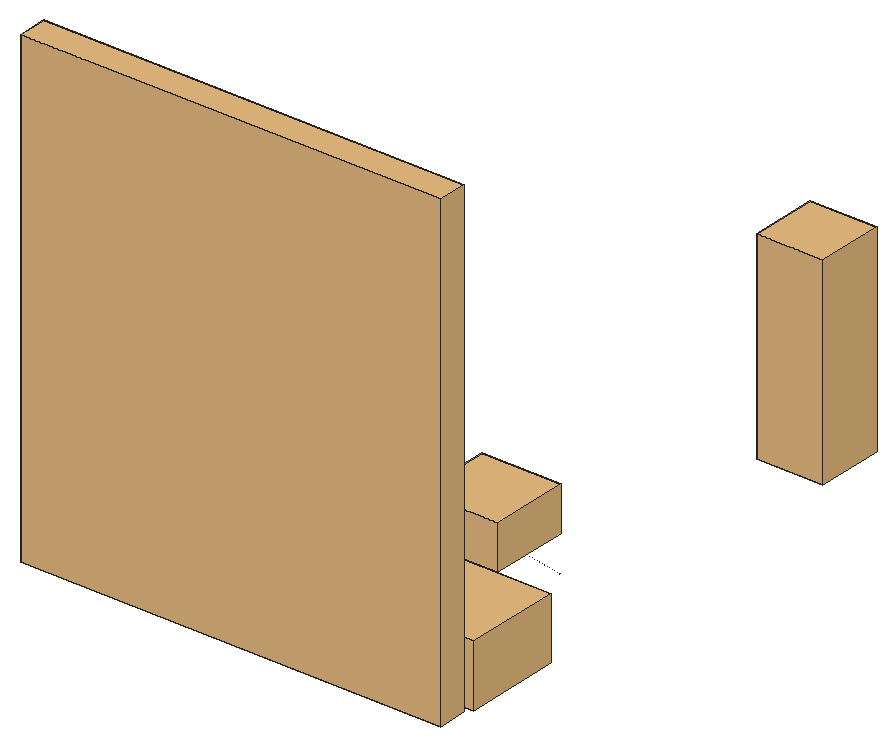
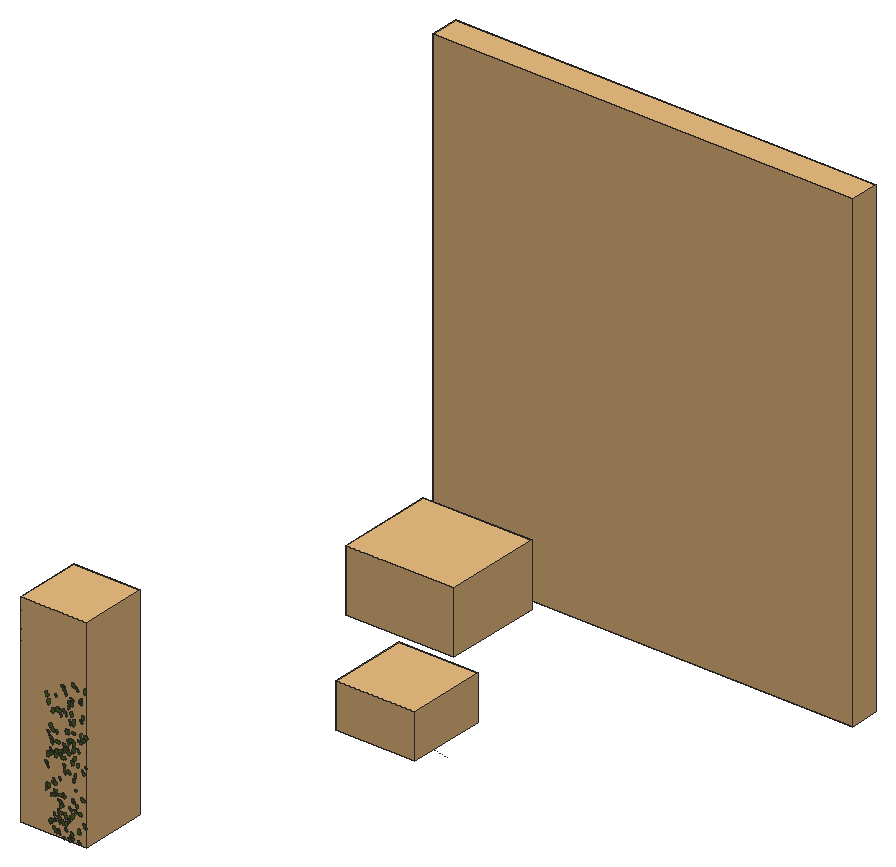
# SketchUp Ruby script. Lengths in inches.
U = 1.inch
M = Sketchup.active_model
def pt(a) = Geom::Point3d.new(a.map { |v| v * U })
def face(e, loops, mat)
  f = e.add_face(loops[0].map { |a| pt(a) })
  loops[1..].each { |l| e.add_face(l.map { |a| pt(a) }).erase! }
  f.material = f.back_material = mat if mat
  f
end
# faces: each face lists its corners as indices into pts; further lists are holes
def faces(e, pts, list, mat = nil) = list.each { |f| face(e, (f[0].is_a?(Array) ? f : [f]).map { |l| l.map { |i| pts[i] } }, mat) }
# xy, xz, yz: faces in a plane at the given z, y or x. An outline is a flat list of corners, or four numbers for a rectangle; further outlines are holes
def ring(l) = l.size == 4 ? [[l[0], l[1]], [l[2], l[1]], [l[2], l[3]], [l[0], l[3]]] : l.each_slice(2).to_a
def flat(e, list, mat, &to3) = list.each { |f| face(e, (f[0].is_a?(Array) ? f : [f]).map { |l| ring(l).map { |u, v| to3.(u, v) } }, mat) }
def xy(e, z, list, mat = nil) = flat(e, list, mat) { |x, y| [x, y, z] }
def xz(e, y, list, mat = nil) = flat(e, list, mat) { |x, z| [x, y, z] }
def yz(e, x, list, mat = nil) = flat(e, list, mat) { |y, z| [x, y, z] }
def lines(e, pts, list) = list.each { |a, b| e.add_line(pt(pts[a]), pt(pts[b])) }
# prism: a flat outline (further loops are holes) pulled along v
def prism(e, loops, v, mat = nil)
  f = face(e, loops, mat); d = Geom::Vector3d.new(v.map { |x| x * U })
  f.pushpull(f.normal.samedirection?(d) ? d.length : -d.length)
end
def box(e, o, s, mat = nil) = prism(e, [[o, [o[0] + s[0], o[1], o[2]], [o[0] + s[0], o[1] + s[1], o[2]], [o[0], o[1] + s[1], o[2]]]], [0, 0, s[2]], mat)
def at(x, y, z, deg = 0) = Geom::Transformation.translation(pt([x, y, z])) * Geom::Transformation.rotation(ORIGIN, Z_AXIS, deg.degrees)
def axes(o, x, y, z) = Geom::Transformation.new([*x, 0, *y, 0, *z, 0, *pt(o).to_a, 1])
def part(name) = M.definitions.add(name)
# library, detail: a bought-in or finely detailed component or shape, given as its bounding box
def library(name, o, s) = part(name).tap { |d| box(d.entities, o, s) }
def detail(e, o, s) = box(e.add_group.entities, o, s)
def put(e, d, t, mat = nil) = e.add_instance(d, t).tap { |i| i.material = mat if mat }
def group(e, t, mat = nil) = e.add_group.tap { |g| g.transformation = t; g.material = mat if mat }.entities
root = M.entities
M.materials.add("[Color M00]1").color = [208, 208, 208]
M.materials.add("[Vegetation Blur 03]").color = [83, 114, 18]
c1 = library("Group\#44",[0,0,-8.125],[130,9,146])
c2 = library("Potted plant",[-17.58,-15.45,-0.53],[33.42,30.09,19.21])
c3 = library("07",[-18.99,-18.99,0],[37.98,37.98,14.32])
c4 = library("Group1\#1",[-13.35,12.45,0],[13.31,13.31,40.49])
c5 = part("ivy")
xy(c5.entities,0,[[0.782,0,0.786,0,0.787,0.005,0.789,0.009,0.821,0.072,0.875,0.147,1.001,0.272,1.073,0.331,1.137,0.363,1.178,0.379,1.223,0.384,1.272,0.383,1.311,0.374,1.36,0.355,1.399,0.334,1.491,0.285,1.541,0.244,1.583,0.199,1.617,0.15,1.64,0.128,1.662,0.115,1.717,0.105,1.745,0.093,1.784,0.054,1.819,0.057,1.854,0.064,1.882,0.075,1.896,0.074,1.91,0.071,1.937,0.063,1.964,0.053,1.99,0.038,2.016,0.015,2.034,0.002,2.04,0,2.038,0.003,2.036,0.007,2.033,0.038,2.036,0.068,2.045,0.1,2.055,0.116,2.064,0.123,2.077,0.129,2.088,0.129,2.106,0.132,2.118,0.13,2.179,0.132,2.207,0.133,2.225,0.133,2.242,0.138,2.22,0.162,2.207,0.186,2.206,0.213,2.212,0.236,2.228,0.262,2.247,0.274,2.298,0.283,2.355,0.294,2.37,0.296,2.376,0.295,2.377,0.3,2.377,0.303,2.385,0.329,2.411,0.37,2.426,0.392,2.449,0.407,2.511,0.426,2.561,0.444,2.619,0.466,2.589,0.469,2.561,0.476,2.501,0.5,2.449,0.516,2.424,0.523,2.401,0.535,2.377,0.556,2.372,0.568,2.36,0.575,2.268,0.586,2.225,0.592,2.207,0.599,2.194,0.61,2.143,0.65,2.13,0.664,2.122,0.682,2.123,0.7,2.13,0.719,2.148,0.75,2.17,0.781,2.195,0.807,2.221,0.828,2.284,0.874,2.291,0.88,2.288,0.887,2.276,0.9,2.267,0.916,2.265,0.933,2.273,0.967,2.292,1.002,2.313,1.03,2.334,1.054,2.348,1.067,2.358,1.074,2.363,1.076,2.362,1.081,2.35,1.094,2.347,1.11,2.35,1.143,2.359,1.18,2.385,1.254,2.415,1.324,2.448,1.393,2.45,1.4,2.446,1.398,2.44,1.394,2.427,1.383,2.402,1.36,2.376,1.339,2.345,1.324,2.305,1.309,2.282,1.303,2.273,1.306,2.245,1.294,2.212,1.287,2.187,1.291,2.163,1.301,2.142,1.316,2.134,1.327,2.124,1.325,2.09,1.292,2.053,1.259,2.014,1.234,1.973,1.215,1.954,1.21,1.931,1.208,1.909,1.212,1.893,1.22,1.879,1.233,1.872,1.248,1.867,1.281,1.864,1.319,1.821,1.258,1.773,1.197,1.726,1.141,1.698,1.121,1.679,1.116,1.666,1.117,1.647,1.122,1.632,1.129,1.62,1.141,1.617,1.154,1.617,1.219,1.621,1.254,1.623,1.268,1.623,1.281,1.618,1.314,1.606,1.346,1.603,1.375,1.607,1.403,1.603,1.467,1.599,1.499,1.605,1.525,1.614,1.552,1.629,1.577,1.635,1.589,1.629,1.587,1.618,1.582,1.596,1.566,1.581,1.556,1.568,1.552,1.557,1.55,1.545,1.553,1.531,1.562,1.522,1.572,1.504,1.591,1.486,1.611,1.474,1.631,1.457,1.666,1.455,1.684,1.457,1.698,1.452,1.715,1.444,1.728,1.424,1.754,1.419,1.772,1.423,1.786,1.434,1.819,1.444,1.848,1.446,1.855,1.44,1.861,1.43,1.867,1.386,1.904,1.349,1.948,1.326,1.973,1.31,1.995,1.288,2.048,1.284,2.153,1.287,2.254,1.284,2.255,1.282,2.253,1.278,2.247,1.274,2.237,1.266,2.216,1.226,2.125,1.208,2.076,1.184,2.033,1.155,1.984,1.135,1.942,1.111,1.899,1.083,1.861,1.053,1.85,1.059,1.83,1.061,1.809,1.056,1.79,1.049,1.767,1.04,1.749,1.018,1.733,0.994,1.726,0.942,1.734,0.95,1.6875,0.944,1.645,0.932,1.608,0.911,1.585,0.881,1.58,0.854,1.582,0.828,1.588,0.785,1.618,0.773,1.625,0.775,1.614,0.779,1.598,0.796,1.502,0.818,1.402,0.861,1.283,0.882,1.224,0.894,1.174,0.892,1.148,0.886,1.123,0.881,1.107,0.872,1.099,0.849,1.094,0.818,1.092,0.789,1.098,0.762,1.107,0.753,1.113,0.721,1.139,0.698,1.163,0.678,1.194,0.665,1.224,0.628,1.28,0.612,1.312,0.606,1.327,0.606,1.314,0.599,1.282,0.594,1.267,0.581,1.256,0.544,1.245,0.512,1.244,0.473,1.249,0.444,1.256,0.382,1.288,0.339,1.306,0.324,1.316,0.317,1.324,0.309,1.326,0.27,1.314,0.227,1.313,0.185,1.3125,0.152,1.317,0.122,1.328,0.092,1.345,0.073,1.353,0.079,1.338,0.092,1.308,0.117,1.249,0.13,1.215,0.139,1.164,0.147,1.148,0.157,1.136,0.163,1.122,0.174,1.086,0.177,1.067,0.182,1.054,0.186,1.043,0.191,1.038,0.211,1.028,0.237,1.005,0.25,0.974,0.253,0.96,0.25,0.944,0.242,0.914,0.243,0.906,0.249,0.902,0.26,0.894,0.289,0.88,0.307,0.873,0.322,0.862,0.364,0.799,0.403,0.738,0.431,0.709,0.439,0.691,0.441,0.678,0.4375,0.66,0.428,0.645,0.394,0.623,0.303,0.594,0.255,0.581,0.214,0.577,0.179,0.573,0.173,0.568,0.175,0.561,0.167,0.55,0.141,0.523,0.113,0.503,0.077,0.49,0.045,0.486,0.026,0.485,0.019,0.486,0.011,0.483,0,0.471,0.014,0.467,0.044,0.455,0.058,0.447,0.07,0.438,0.097,0.411,0.125,0.394,0.158,0.377,0.174,0.366,0.182,0.359,0.185,0.361,0.242,0.331,0.253,0.316,0.258,0.303,0.262,0.283,0.274,0.278,0.308,0.274,0.341,0.252,0.366,0.226,0.366,0.222,0.37,0.22,0.38,0.221,0.395,0.221,0.425,0.216,0.45,0.207,0.465,0.192,0.473,0.178,0.484,0.15,0.489,0.116,0.483,0.089,0.468,0.058,0.45,0.035,0.435,0.018,0.429,0.011,0.434,0.012,0.438,0.014,0.469,0.019,0.542,0.016,0.581,0.015,0.612,0.027,0.68,0.055,0.696,0.057,0.712,0.052,0.73,0.045,0.741,0.036,0.766,0.014]])
p = [[115.39,75.31,5.05],[115.39,75.31,5],[115.4,75.3125,5.03],[84.96,81.43,5],[84.97,81.43,5.03],[84.04,81.61,5.03],
  [84.05,81.61,5],[84.03,81.62,5],[84.98,81.43,5],[85.88,81.24,5],[85.89,81.24,5.03],[85.9,81.24,5],
  [79.43,82.54,5.03],[79.44,82.54,5],[80.34,82.36,5],[80.35,82.35,5.03],[80.36,82.35,5],[79.42,82.54,5],
  [81.27,82.17,5],[81.28,82.17,5.03],[83.11,81.8,5],[83.12,81.8,5.03],[83.13,81.8,5],[82.2,81.98,5.03],
  [82.21,81.98,5],[81.29,82.17,5],[82.19,81.99,5],[86.8,81.06,5],[86.8125,81.06,5.03],[86.82,81.06,5],
  [74.8125,83.47,5],[74.82,83.47,5.03],[74.83,83.46,5],[75.73,83.28,5],[75.74,83.28,5.03],[75.75,83.28,5],
  [76.66,83.1,5.03],[76.67,83.09,5],[76.66,83.1,5],[77.58,82.91,5],[77.59,82.91,5.03],[77.6,82.91,5],
  [78.51,82.73,5.03],[78.52,82.72,5],[78.5,82.73,5],[90.5,80.32,5.03],[90.51,80.3125,5],[87.72,80.875,5],
  [87.73,80.87,5.03],[89.58,80.5,5.03],[89.59,80.5,5],[90.49,80.32,5],[88.65,80.6875,5],[88.66,80.6875,5.03],
  [89.57,80.5,5],[87.74,80.87,5],[88.67,80.69,5],[94.19,79.58,5.03],[94.2,79.57,5],[92.34,79.95,5],
  [92.35,79.95,5.03],[91.41,80.13,5],[91.42,80.13,5.03],[93.27,79.76,5.03],[93.28,79.76,5],[93.26,79.76,5],
  [92.35,79.94,5],[91.43,80.13,5],[94.18,79.58,5],[95.11,79.39,5.03],[95.12,79.39,5],[96.03,79.21,5],
  [96.03,79.2,5.03],[96.04,79.2,5],[97.87,78.84,5],[97.88,78.83,5.03],[95.1,79.39,5],[96.95,79.02,5],
  [96.96,79.02,5.03],[96.97,79.02,5],[98.79,78.65,5],[98.8,78.65,5.03],[98.8125,78.65,5],[97.89,78.83,5],
  [99.72,78.46,5.03],[99.73,78.46,5],[100.64,78.28,5],[100.65,78.28,5.03],[100.66,78.28,5],[99.71,78.47,5],
  [101.56,78.09,5],[101.57,78.09,5.03],[102.49,77.91,5.03],[102.5,77.91,5],[103.41,77.72,5.03],[103.42,77.72,5],
  [104.33,77.54,5],[104.34,77.54,5.03],[101.58,78.09,5],[104.35,77.53,5],[103.4,77.72,5],[102.48,77.91,5],
  [107.1,76.98,5.03],[107.11,76.98,5],[106.18,77.17,5.03],[106.19,77.16,5],[105.26,77.35,5.03],[105.27,77.35,5],
  [108.02,76.8,5],[108.03,76.8,5.03],[105.25,77.35,5],[108.03,76.79,5],[107.09,76.98,5],[106.17,77.17,5],
  [110.79,76.24,5.03],[110.8,76.24,5],[108.9375,76.61,5],[108.95,76.61,5.03],[109.87,76.42,5.03],[109.88,76.42,5],
  [111.71,76.05,5.03],[111.72,76.05,5],[111.71,76.06,5],[110.78,76.24,5],[109.86,76.43,5],[108.96,76.61,5],
  [112.63,75.87,5],[112.64,75.87,5.03],[112.65,75.87,5],[113.56,75.68,5.03],[113.57,75.68,5],[113.55,75.6875,5],
  [114.47,75.5,5],[114.48,75.5,5.03],[114.49,75.5,5],[115.41,75.3125,5]]
faces(root,p,[[0,1,2]])
lines(root,p,[[3,4],[5,6],[7,5],[4,8],[9,10],[10,11],[12,13],[14,15],[15,16],[17,12],[18,19],[20,21],
  [21,22],[23,24],[19,25],[26,23],[27,28],[28,29],[30,31],[31,32],[33,34],[34,35],[36,37],[38,36],
  [39,40],[40,41],[42,43],[44,42],[45,46],[47,48],[49,50],[51,45],[52,53],[54,49],[48,55],[53,56],
  [57,58],[59,60],[61,62],[63,64],[65,63],[60,66],[62,67],[68,57],[69,70],[71,72],[72,73],[74,75],
  [76,69],[77,78],[78,79],[80,81],[81,82],[75,83],[84,85],[86,87],[87,88],[89,84],[90,91],[92,93],
  [94,95],[96,97],[91,98],[97,99],[100,94],[101,92],[102,103],[104,105],[106,107],[108,109],[110,106],[109,111],
  [112,102],[113,104],[114,115],[116,117],[118,119],[120,121],[122,120],[123,114],[124,118],[117,125],[126,127],[127,128],
  [129,130],[131,129],[132,133],[133,134],[2,135]])
put(root,c1,at(9,0,12.125))
put(root,c2,at(123.79,27.2,4))
put(root,c3,axes([91.58,78.16,5.375],[0.64,0,0],[0,0.64,0],[0,0,0.96]))
put(root,c4,axes([136.72,131.48,4],[1.54,0,0],[0,1.54,0],[0,0,1.54]),"[Color M00]1")
put(root,c5,axes([116.45,173.8,31.39],[0.62306,-0.44776,0.08452],[0.0504,-0.33563,-0.52711],[-0.23565,-1.25564,0.11075]),"[Vegetation Blur 03]")
put(root,c5,axes([120.39,173.8,24.18],[0.48124,-0.36893,0.30519],[0.35516,-0.24188,-0.41903],[-0.21409,-1.23057,-0.00913]),"[Vegetation Blur 03]")
put(root,c5,axes([125.86,173.8,24.21],[0.50493,-0.24622,0.19162],[0.19585,-0.34808,-0.41408],[-0.17632,-1.09173,0.08881]),"[Vegetation Blur 03]")
put(root,c5,axes([124.47,173.8,28.85],[0.61028,-0.27277,0.17175],[0.18054,-0.30337,-0.50308],[-0.17106,-1.2933,0.08178]),"[Vegetation Blur 03]")
put(root,c5,axes([119.33,173.8,32.88],[0.58162,-0.37165,0.13863],[0.15197,-0.16988,-0.49633],[-0.1959,-1.23523,0.02655]),"[Vegetation Blur 03]")
put(root,c5,axes([122.09,173.8,6.63],[0.29467,-0.10714,0.44848],[0.50944,-0.44068,-0.23951],[-0.21249,-1.20507,0.04772]),"[Vegetation Blur 03]")
put(root,c5,axes([117.66,173.8,38.14],[0.18149,-0.29755,0.51892],[0.63719,-0.20751,-0.16715],[-0.13848,-1.34475,-0.08903]),"[Vegetation Blur 03]")
put(root,c5,axes([120.04,173.8,35.1875],[0.25712,-0.18798,0.42224],[0.4923,-0.32764,-0.22263],[-0.18343,-1.14283,-0.00563]),"[Vegetation Blur 03]")
put(root,c5,axes([114.12,173.8,48.42],[0.47356,-0.40672,0.26845],[0.33871,-0.06229,-0.41283],[-0.18036,-1.18486,-0.07045]),"[Vegetation Blur 03]")
put(root,c5,axes([118.28,173.8,7.04],[0.3696,-0.27711,0.38105],[0.45779,-0.2062,-0.31935],[-0.16294,-1.2079,-0.0329]),"[Vegetation Blur 03]")
put(root,c5,axes([119.99,173.8,11.98],[0.55958,-0.3731,0.26041],[0.3198,-0.09162,-0.47837],[-0.18004,-1.32239,-0.04033]),"[Vegetation Blur 03]")
put(root,c5,axes([119.22,173.8,15.21],[0.5074,-0.4678,-0.2898],[-0.37384,0.02954,-0.44347],[-0.19497,-1.27408,0.09613]),"[Vegetation Blur 03]")
put(root,c5,axes([118.19,173.8,45.25],[0.5878,-0.24093,0.03931],[0.02588,-0.23212,-0.48155],[-0.12393,-1.19122,0.08588]),"[Vegetation Blur 03]")
put(root,c5,axes([115.75,173.8,44.97],[0.11866,-0.26117,0.39663],[0.48542,-0.20436,-0.1179],[-0.12904,-1.00894,-0.07879]),"[Vegetation Blur 03]")
put(root,c5,axes([114.48,173.8,25.76],[0.52711,-0.21147,0.33505],[0.39283,-0.25745,-0.4372],[-0.15742,-1.35053,0.03088]),"[Vegetation Blur 03]")
put(root,c5,axes([121.64,173.8,27.84],[0.18528,-0.05644,0.53215],[0.61865,-0.42892,-0.15063],[-0.2078,-1.32731,0.02605]),"[Vegetation Blur 03]")
put(root,c5,axes([116.65,173.8,48.48],[0.53111,-0.22481,0.11811],[0.12292,-0.23121,-0.43739],[-0.1333,-1.10892,0.06725]),"[Vegetation Blur 03]")
put(root,c5,axes([117.65,173.8,33.41],[0.62179,-0.3866,0.07255],[0.08725,-0.03824,-0.53009],[-0.18864,-1.29198,-0.00602]),"[Vegetation Blur 03]")
put(root,c5,axes([118.99,173.8,11.69],[0.16819,-0.22664,0.32974],[0.39401,-0.21788,-0.15742],[-0.14187,-0.87383,-0.04627]),"[Vegetation Blur 03]")
put(root,c5,axes([121.23,173.8,15.18],[0.5531,-0.30937,0.07702],[0.082,-0.11827,-0.46698],[-0.15743,-1.14854,0.02734]),"[Vegetation Blur 03]")
put(root,c5,axes([121.57,173.8,14.93],[0.62192,-0.51222,0.08279],[0.13225,0.12501,-0.54004],[-0.23401,-1.29066,-0.08517]),"[Vegetation Blur 03]")
put(root,c5,axes([117.16,173.8,14.91],[0.58633,-0.27865,-0.1062],[-0.1477,-0.14213,-0.48453],[-0.11598,-1.22771,0.08019]),"[Vegetation Blur 03]")
put(root,c5,axes([114.79,173.8,35.28],[0.64635,-0.1795,-0.0483],[-0.07498,-0.25102,-0.52154],[-0.0741,-1.31182,0.10641]),"[Vegetation Blur 03]")
put(root,c5,axes([119.3125,173.8,35.25],[0.21062,-0.15839,0.41958],[0.49728,-0.27124,-0.18238],[-0.15148,-1.11064,-0.0153]),"[Vegetation Blur 03]")
put(root,c5,axes([123.64,173.8,17.2],[0.43914,-0.29657,0.03896],[0.03337,-0.10478,-0.37595],[-0.14811,-0.90294,0.03083]),"[Vegetation Blur 03]")
put(root,c5,axes([115.8,173.8,35.73],[0.12614,-0.2409,0.28031],[0.3435,-0.16191,-0.12485],[-0.11696,-0.73532,-0.06434]),"[Vegetation Blur 03]")
put(root,c5,axes([125.49,173.8,41.39],[0.07798,-0.22712,0.49701],[0.61066,-0.17712,-0.07655],[-0.10063,-1.25091,-0.0794]),"[Vegetation Blur 03]")
put(root,c5,axes([125.76,173.8,44.07],[0.58958,-0.29849,0.19052],[0.22934,-0.09222,-0.49546],[-0.15145,-1.30163,-0.00859]),"[Vegetation Blur 03]")
put(root,c5,axes([122.16,173.8,12.37],[0.33688,-0.08622,0.33874],[0.38873,-0.33347,-0.27086],[-0.15137,-1.04826,0.0583]),"[Vegetation Blur 03]")
put(root,c5,axes([121.27,173.8,48.4],[0.54958,-0.28156,-0.28314],[-0.3622,-0.10008,-0.45262],[-0.08884,-1.33367,0.09374]),"[Vegetation Blur 03]")
put(root,c5,axes([120.13,173.8,8.6],[0.49081,-0.25055,0.00673],[-0.00728,-0.13032,-0.40947],[-0.12182,-1.0017,0.05159]),"[Vegetation Blur 03]")
put(root,c5,axes([114.69,173.8,40.7],[0.32628,-0.20206,0.40603],[0.49033,-0.18475,-0.27691],[-0.12932,-1.21026,-0.02552]),"[Vegetation Blur 03]")
put(root,c5,axes([118.06,173.8,16.98],[0.30081,-0.15518,0.1985],[0.21889,-0.23826,-0.25024],[-0.13012,-0.75955,0.03794]),"[Vegetation Blur 03]")
put(root,c5,axes([115.91,173.8,6.41],[0.52824,-0.2088,0.07813],[0.0803,-0.17577,-0.43551],[-0.11407,-1.09065,0.05523]),"[Vegetation Blur 03]")
put(root,c5,axes([124.375,173.8,17.54],[0.50163,-0.24569,-0.26541],[-0.34021,-0.12729,-0.40976],[-0.06534,-1.2236,0.09592]),"[Vegetation Blur 03]")
put(root,c5,axes([114.32,173.8,11.27],[0.44114,-0.2833,-0.10477],[-0.14493,-0.08165,-0.37173],[-0.12012,-0.94191,0.06374]),"[Vegetation Blur 03]")
put(root,c5,axes([118.9,173.8,6.19],[0.53858,-0.252,0.05397],[0.05479,-0.1161,-0.44944],[-0.12794,-1.11057,0.03474]),"[Vegetation Blur 03]")
put(root,c5,axes([123.18,173.8,16.97],[0.15407,-0.1087,0.33806],[0.39127,-0.27976,-0.13293],[-0.14585,-0.86534,0.00051]),"[Vegetation Blur 03]")
put(root,c5,axes([119.56,173.8,11.26],[0.4884,-0.38994,-0.09349],[-0.11293,0.05241,-0.42733],[-0.19047,-1.03097,0.01363]),"[Vegetation Blur 03]")
put(root,c5,axes([123.17,173.8,32.56],[0.49181,-0.15671,-0.3315],[-0.41314,-0.21702,-0.39213],[0.00973,-1.29451,0.10587]),"[Vegetation Blur 03]")
put(root,c5,axes([120.17,173.8,31.01],[0.44605,-0.17185,0.11357],[0.12178,-0.19918,-0.36599],[-0.10728,-0.94065,0.05675]),"[Vegetation Blur 03]")
put(root,c5,axes([117.75,173.8,30.62],[0.10022,-0.2222,0.4688],[0.57871,-0.13035,-0.09212],[-0.08191,-1.19279,-0.07727]),"[Vegetation Blur 03]")
put(root,c5,axes([122.02,173.8,21.9],[0.3651,-0.20886,0.13721],[0.15459,-0.14475,-0.30864],[-0.12111,-0.81437,0.01967]),"[Vegetation Blur 03]")
put(root,c5,axes([122.89,173.8,6.98],[0.51611,-0.14167,0.29822],[0.35265,-0.22138,-0.42305],[-0.1179,-1.28232,0.04009]),"[Vegetation Blur 03]")
put(root,c5,axes([117.24,173.8,23.81],[0.1731,-0.14266,0.38005],[0.45428,-0.21748,-0.15066],[-0.12362,-0.99891,-0.02148]),"[Vegetation Blur 03]")
put(root,c5,axes([124.01,173.8,39.72],[0.30187,-0.29092,0.34167],[0.43037,-0.04293,-0.25902],[-0.10016,-1.06123,-0.08319]),"[Vegetation Blur 03]")
put(root,c5,axes([121.5625,173.8,39.49],[0.34266,-0.16677,0.2483],[0.29126,-0.18349,-0.28712],[-0.11956,-0.92493,0.01219]),"[Vegetation Blur 03]")
put(root,c5,axes([122.13,173.8,11.41],[0.56213,-0.17838,-0.00831],[-0.02255,-0.16495,-0.45927],[-0.08432,-1.14512,0.06745]),"[Vegetation Blur 03]")
put(root,c5,axes([117.71,173.8,16.9],[0.37075,-0.20222,0.27738],[0.33431,-0.13128,-0.31269],[-0.11578,-1.02663,-0.01465]),"[Vegetation Blur 03]")
put(root,c5,axes([123.77,173.8,20.86],[0.29156,-0.09126,0.22735],[0.25627,-0.25873,-0.23525],[-0.11785,-0.78843,0.05088]),"[Vegetation Blur 03]")
put(root,c5,axes([119.98,173.8,9.65],[0.28606,-0.20547,0.36321],[0.44363,-0.1257,-0.24391],[-0.10592,-1.08138,-0.04066]),"[Vegetation Blur 03]")
put(root,c5,axes([118.26,173.8,44.08],[0.56579,-0.26175,0.06944],[0.08066,-0.05979,-0.47321],[-0.13005,-1.17586,0.0086]),"[Vegetation Blur 03]")
put(root,c5,axes([117.95,173.8,6.4],[0.19741,-0.09695,0.50499],[0.60705,-0.24693,-0.16553],[-0.12869,-1.3135,-0.00615]),"[Vegetation Blur 03]")
put(root,c5,axes([116.46,173.8,27.2],[0.23432,-0.21265,0.28086],[0.3439,-0.11223,-0.20448],[-0.10411,-0.84934,-0.0433]),"[Vegetation Blur 03]")
put(root,c5,axes([118.07,173.8,12.14],[0.09309,-0.2572,0.47512],[0.59358,-0.05541,-0.08218],[-0.0469,-1.21192,-0.09707]),"[Vegetation Blur 03]")
put(root,c5,axes([124.92,173.8,32.05],[0.48032,-0.40321,-0.3461],[-0.42858,0.11763,-0.41773],[-0.18586,-1.31325,0.06885]),"[Vegetation Blur 03]")
put(root,c5,axes([115.86,173.8,45.49],[0.45619,-0.27219,-0.21417],[-0.27378,-0.03129,-0.38217],[-0.10679,-1.08253,0.0649]),"[Vegetation Blur 03]")
put(root,c5,axes([123.4375,173.8,10.15],[0.27567,-0.18278,0.07916],[0.08,-0.13493,-0.23455],[-0.1044,-0.58604,0.02931]),"[Vegetation Blur 03]")
put(root,c5,axes([119.24,173.8,42.58],[0.31604,-0.28517,0.16056],[0.20748,-0.01555,-0.27638],[-0.12189,-0.7659,-0.05417]),"[Vegetation Blur 03]")
put(root,c5,axes([117.7,173.8,48.87],[0.27432,-0.11887,0.39101],[0.46845,-0.2067,-0.22879],[-0.11587,-1.1171,0.00072]),"[Vegetation Blur 03]")
put(root,c5,axes([120.43,173.8,46.66],[0.3032,0.00804,0.42723],[0.50376,-0.343,-0.23711],[-0.14236,-1.19666,0.07083]),"[Vegetation Blur 03]")
put(root,c5,axes([115.36,173.8,45.6],[0.40522,-0.15446,0.13943],[0.15914,-0.15283,-0.3347],[-0.09744,-0.89194,0.0332]),"[Vegetation Blur 03]")
put(root,c5,axes([118.2,173.8,41.15],[0.5598,-0.34639,0.09978],[0.13771,0.07562,-0.47332],[-0.15594,-1.17668,-0.05979]),"[Vegetation Blur 03]")
put(root,c5,axes([115.29,173.8,39.72],[0.34108,-0.07651,0.26436],[0.30846,-0.23678,-0.27587],[-0.10562,-0.93855,0.04805]),"[Vegetation Blur 03]")
put(root,c5,axes([117.45,173.8,28.49],[0.13916,-0.21976,0.37305],[0.46529,-0.06512,-0.12164],[-0.06205,-0.98109,-0.07549]),"[Vegetation Blur 03]")
put(root,c5,axes([120.95,173.8,6.27],[0.36884,-0.18268,-0.08765],[-0.12074,-0.10682,-0.30338],[-0.06956,-0.78327,0.06182]),"[Vegetation Blur 03]")
put(root,c5,axes([119.09,173.8,11.24],[0.27201,-0.08351,0.1346],[0.14493,-0.22002,-0.21655],[-0.08857,-0.61651,0.05905]),"[Vegetation Blur 03]")
put(root,c5,axes([115.59,173.8,9.01],[0.44693,-0.21309,0.34937],[0.42945,-0.06761,-0.37241],[-0.09772,-1.27172,-0.03874]),"[Vegetation Blur 03]")
put(root,c5,axes([124.81,173.8,32.5],[0.35673,-0.12377,0.22075],[0.25958,-0.16822,-0.29423],[-0.09696,-0.90576,0.02448]),"[Vegetation Blur 03]")
put(root,c5,axes([115.39,173.8,34.33],[0.60257,-0.08021,0.1387],[0.16152,-0.21723,-0.48713],[-0.06569,-1.26991,0.07457]),"[Vegetation Blur 03]")
put(root,c5,axes([120.01,173.8,30.02],[0.0827,-0.23642,0.52033],[0.64705,-0.03418,-0.07095],[-0.03151,-1.3225,-0.09118]),"[Vegetation Blur 03]")
put(root,c5,axes([117.64,173.8,22.84],[0.37427,-0.16845,0.18276],[0.21743,-0.11081,-0.31265],[-0.09784,-0.89065,0.00433]),"[Vegetation Blur 03]")
put(root,c5,axes([122.64,173.8,30.18],[0.08303,-0.1967,-0.5076],[-0.62878,-0.07669,-0.06383],[0.02474,-1.28895,0.08126]),"[Vegetation Blur 03]")
put(root,c5,axes([122.94,173.8,34.79],[0.45964,-0.254,0.03008],[0.03689,-0.00973,-0.3884],[-0.12342,-0.94883,-0.00407]),"[Vegetation Blur 03]")
put(root,c5,axes([124.56,173.8,10.22],[0.52518,-0.29878,-0.23016],[-0.2856,0.04291,-0.44284],[-0.13799,-1.22592,0.0406]),"[Vegetation Blur 03]")
put(root,c5,axes([120.22,173.8,41.1],[0.56013,-0.13091,0.22183],[0.26451,-0.15182,-0.45897],[-0.08921,-1.27215,0.03195]),"[Vegetation Blur 03]")
put(root,c5,axes([126.29,173.8,18.86],[0.1642,-0.18374,0.20113],[0.24769,-0.08699,-0.14719],[-0.08574,-0.60314,-0.04004]),"[Vegetation Blur 03]")
put(root,c5,axes([121.96,173.8,40.88],[0.47833,-0.24749,0.17674],[0.22101,-0.01127,-0.40089],[-0.11188,-1.08043,-0.0363]),"[Vegetation Blur 03]")
put(root,c5,axes([123.52,173.8,20.72],[0.62885,-0.10059,-0.07918],[-0.103,-0.17922,-0.50906],[-0.03454,-1.29703,0.07648]),"[Vegetation Blur 03]")
put(root,c5,axes([118.8,173.8,34.3],[0.50454,-0.20666,-0.19788],[-0.2502,-0.0525,-0.4163],[-0.0792,-1.15072,0.05453]),"[Vegetation Blur 03]")
put(root,c5,axes([118.9,173.8,30.11],[0.57292,-0.29787,0.17247],[0.22282,0.05394,-0.47834],[-0.12636,-1.25544,-0.06147]),"[Vegetation Blur 03]")
put(root,c5,axes([126.05,173.8,25.33],[0.43109,-0.16307,0.09857],[0.11374,-0.09903,-0.3571],[-0.08905,-0.91592,0.02106]),"[Vegetation Blur 03]")
put(root,c5,axes([123.43,173.8,18.61],[0.48596,-0.138,-0.11802],[-0.15256,-0.12597,-0.39525],[-0.04619,-1.03571,0.0638]),"[Vegetation Blur 03]")
put(root,c5,axes([124.31,173.8,31.85],[0.25768,-0.12141,0.16925],[0.19637,-0.14245,-0.21521],[-0.08903,-0.66558,0.01519]),"[Vegetation Blur 03]")
put(root,c5,axes([124.82,173.8,27.65],[0.09017,-0.06413,0.35822],[0.42718,-0.20848,-0.07749],[-0.10559,-0.89821,-0.00759]),"[Vegetation Blur 03]")
put(root,c5,axes([120.6875,173.8,32.09],[0.442,-0.16404,-0.03453],[-0.05057,-0.08968,-0.36412],[-0.07475,-0.90929,0.04214]),"[Vegetation Blur 03]")
put(root,c5,axes([121.91,173.8,18.2],[0.52837,-0.04737,-0.26503],[-0.32337,-0.22367,-0.42312],[0.03764,-1.25647,0.08531]),"[Vegetation Blur 03]")
put(root,c5,axes([114.11,173.8,11.66],[0.54065,-0.21536,0.14176],[0.17436,-0.02611,-0.44914],[-0.10356,-1.16826,-0.01609]),"[Vegetation Blur 03]")
put(root,c5,axes([123.8,173.8,34.52],[0.31957,-0.02324,0.46113],[0.55443,-0.24575,-0.25788],[-0.10943,-1.31297,0.04011]),"[Vegetation Blur 03]")
put(root,c5,axes([125.33,173.8,27.72],[0.52923,-0.27231,0.14829],[0.19148,0.04522,-0.44212],[-0.11773,-1.15056,-0.05247]),"[Vegetation Blur 03]")
put(root,c5,axes([122.09,173.8,13.21],[0.5099,-0.05447,-0.26558],[-0.32487,-0.20771,-0.40876],[0.03235,-1.22728,0.08097]),"[Vegetation Blur 03]")
put(root,c5,axes([123.3,173.8,44.57],[0.32682,-0.209,0.08086],[0.0994,-0.02803,-0.27901],[-0.10124,-0.70219,-0.01293]),"[Vegetation Blur 03]")
put(root,c5,axes([114.08,173.8,27.76],[0.29106,-0.10296,0.03164],[0.02588,-0.14904,-0.23485],[-0.05776,-0.58557,0.05421]),"[Vegetation Blur 03]")
put(root,c5,axes([117.24,173.8,20.64],[0.31975,-0.13436,-0.03342],[-0.05173,-0.10756,-0.26163],[-0.05713,-0.65457,0.04985]),"[Vegetation Blur 03]")
put(root,c5,axes([119.3,173.8,43.92],[0.22551,-0.17157,0.19026],[0.23404,-0.06401,-0.19384],[-0.08079,-0.66437,-0.03046]),"[Vegetation Blur 03]")
put(root,c5,axes([122.13,173.8,16.16],[0.41492,-0.08686,-0.03354],[-0.04844,-0.1605,-0.33372],[-0.03354,-0.84286,0.067]),"[Vegetation Blur 03]")
put(root,c5,axes([116.125,173.8,14.86],[0.33179,-0.22508,-0.3253],[-0.40723,0.00189,-0.27687],[-0.0707,-1.0672,0.06812]),"[Vegetation Blur 03]")
put(root,c5,axes([122.7,173.8,29.14],[0.40671,-0.14437,0.24599],[0.29835,-0.08915,-0.33679],[-0.0822,-1.03788,-0.00529]),"[Vegetation Blur 03]")
put(root,c5,axes([124.76,173.8,16.33],[0.10915,-0.09215,0.23401],[0.27778,-0.14927,-0.09555],[-0.08399,-0.61343,-0.0119]),"[Vegetation Blur 03]")
put(root,c5,axes([121.53,173.8,28.7],[0.25465,-0.11048,-0.36792],[-0.45313,-0.12762,-0.20287],[0.02807,-1.05778,0.0629]),"[Vegetation Blur 03]")
put(root,c5,axes([124.92,173.8,35.4],[0.10455,-0.16948,0.36645],[0.45413,-0.0579,-0.09052],[-0.04648,-0.94693,-0.06005]),"[Vegetation Blur 03]")
put(root,c5,axes([114.9,173.8,36.65],[0.1603,-0.20672,-0.46475],[-0.57787,-0.01388,-0.13179],[-0.02063,-1.21728,0.08043]),"[Vegetation Blur 03]")
put(root,c5,axes([122.88,173.8,28.36],[0.58972,-0.25941,0.10506],[0.13617,0.04808,-0.49046],[-0.11798,-1.24117,-0.04096]),"[Vegetation Blur 03]")
put(root,c5,axes([118.79,173.8,38.21],[0.29872,-0.15455,0.15212],[0.18312,-0.07365,-0.25129],[-0.08276,-0.72081,-0.00694]),"[Vegetation Blur 03]")
put(root,c5,axes([126,173.8,34.34],[0.30417,-0.25351,-0.27604],[-0.3464,0.04167,-0.26026],[-0.0979,-0.93513,0.06323]),"[Vegetation Blur 03]")
put(root,c5,axes([124.875,173.8,8.72],[0.09186,-0.01547,0.40746],[0.48625,-0.23456,-0.07442],[-0.11344,-1.01793,0.01096]),"[Vegetation Blur 03]")
put(root,c5,axes([118.05,173.8,7.93],[0.51714,-0.23527,0.06533],[0.0842,0.02179,-0.43163],[-0.1113,-1.07662,-0.02301]),"[Vegetation Blur 03]")
put(root,c5,axes([120.72,173.8,30.17],[0.49069,-0.15556,0.05335],[0.06086,-0.06942,-0.40473],[-0.07927,-1.0163,0.01948]),"[Vegetation Blur 03]")
put(root,c5,axes([117.6,173.8,36.3125],[0.49447,-0.06651,0.04707],[0.05156,-0.17262,-0.39913],[-0.04138,-1.00977,0.06513]),"[Vegetation Blur 03]")
put(root,c5,axes([121.11,173.8,10.47],[0.46353,-0.32199,-0.04056],[-0.03174,0.12476,-0.39742],[-0.16108,-0.95117,-0.0384]),"[Vegetation Blur 03]")
put(root,c5,axes([117.97,173.8,27.97],[0.56984,-0.3114,0.00181],[0.01697,0.11385,-0.47886],[-0.15039,-1.16708,-0.04719]),"[Vegetation Blur 03]")
put(root,c5,axes([126.14,173.8,17.92],[0.34195,-0.22556,0.12659],[0.16367,0.01646,-0.28987],[-0.09636,-0.7725,-0.04314]),"[Vegetation Blur 03]")
put(root,c5,axes([120.32,173.8,17.4375],[0.45366,-0.05419,0.38117],[0.46073,-0.18,-0.36926],[-0.08098,-1.3277,0.0345]),"[Vegetation Blur 03]")
put(root,c5,axes([120.02,173.8,40.34],[0.3125,-0.15896,0.12959],[0.15654,-0.05797,-0.26261],[-0.08171,-0.71898,-0.00748]),"[Vegetation Blur 03]")
put(root,c5,axes([122.2,173.8,10.1],[0.29646,-0.18293,-0.03481],[-0.04858,-0.02904,-0.25162],[-0.08579,-0.61566,0.02221]),"[Vegetation Blur 03]")
put(root,c5,axes([119.69,173.8,25.4375],[0.39569,-0.25539,-0.40505],[-0.50198,0.05522,-0.33211],[-0.09868,-1.305,0.06522]),"[Vegetation Blur 03]")
put(root,c5,axes([123.79,173.8,11.625],[0.27556,-0.19726,0.13683],[0.17351,-0.01114,-0.23526],[-0.08482,-0.66366,-0.03672]),"[Vegetation Blur 03]")
put(root,c5,axes([120.1,173.8,46.1],[0.3345,-0.16348,0.07359],[0.08724,-0.0471,-0.28058],[-0.08265,-0.71135,0.00167]),"[Vegetation Blur 03]")
put(root,c5,axes([122.66,173.8,41.0625],[0.39765,-0.2594,0.13842],[0.18466,0.06494,-0.33421],[-0.10274,-0.88724,-0.06493]),"[Vegetation Blur 03]")
put(root,c5,axes([123.35,173.8,7.21],[0.24806,0.03915,0.43187],[0.51673,-0.28046,-0.19369],[-0.11561,-1.16947,0.06091]),"[Vegetation Blur 03]")
put(root,c5,axes([116.68,173.8,15.54],[0.07106,0.03212,0.39333],[0.4647,-0.27217,-0.05243],[-0.12873,-0.96482,0.02788]),"[Vegetation Blur 03]")
put(root,c5,axes([125.18,173.8,18.79],[0.32691,-0.16543,0.24576],[0.30294,-0.04245,-0.2729],[-0.07327,-0.91364,-0.03182]),"[Vegetation Blur 03]")
put(root,c5,axes([121.14,173.8,26.7],[0.28967,-0.12811,-0.2275],[-0.2852,-0.08534,-0.23432],[-0.01552,-0.82284,0.05972]),"[Vegetation Blur 03]")
put(root,c5,axes([118.84,173.8,39.01],[0.33002,-0.10362,0.05882],[0.06392,-0.11285,-0.27012],[-0.06037,-0.68589,0.03556]),"[Vegetation Blur 03]")
put(root,c5,axes([114.59,173.8,18.79],[0.61675,-0.12461,0.11294],[0.13479,-0.08629,-0.50526],[-0.06818,-1.29784,0.02275]),"[Vegetation Blur 03]")
